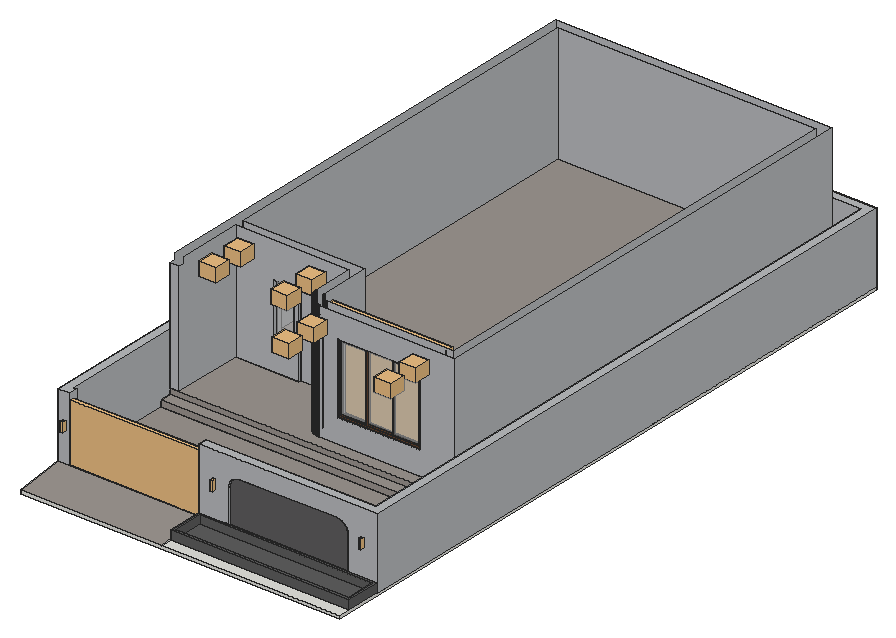
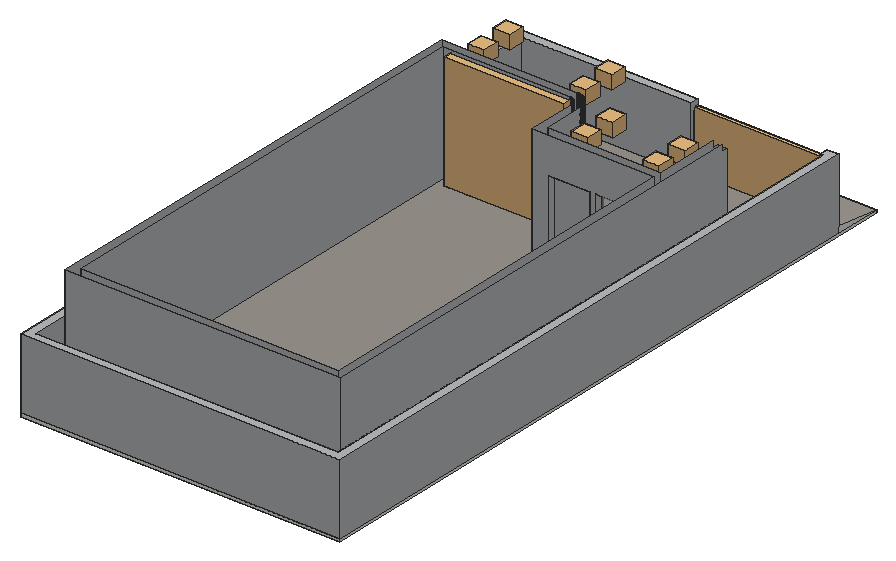
# SketchUp Ruby script. Lengths in inches.
U = 1.inch
M = Sketchup.active_model
def pt(a) = Geom::Point3d.new(a.map { |v| v * U })
def face(e, loops, mat)
  f = e.add_face(loops[0].map { |a| pt(a) })
  loops[1..].each { |l| e.add_face(l.map { |a| pt(a) }).erase! }
  f.material = f.back_material = mat if mat
  f
end
# faces: each face lists its corners as indices into pts; further lists are holes
def faces(e, pts, list, mat = nil) = list.each { |f| face(e, (f[0].is_a?(Array) ? f : [f]).map { |l| l.map { |i| pts[i] } }, mat) }
# xy, xz, yz: faces in a plane at the given z, y or x. An outline is a flat list of corners, or four numbers for a rectangle; further outlines are holes
def ring(l) = l.size == 4 ? [[l[0], l[1]], [l[2], l[1]], [l[2], l[3]], [l[0], l[3]]] : l.each_slice(2).to_a
def flat(e, list, mat, &to3) = list.each { |f| face(e, (f[0].is_a?(Array) ? f : [f]).map { |l| ring(l).map { |u, v| to3.(u, v) } }, mat) }
def xy(e, z, list, mat = nil) = flat(e, list, mat) { |x, y| [x, y, z] }
def xz(e, y, list, mat = nil) = flat(e, list, mat) { |x, z| [x, y, z] }
def yz(e, x, list, mat = nil) = flat(e, list, mat) { |y, z| [x, y, z] }
def lines(e, pts, list) = list.each { |a, b| e.add_line(pt(pts[a]), pt(pts[b])) }
# prism: a flat outline (further loops are holes) pulled along v
def prism(e, loops, v, mat = nil)
  f = face(e, loops, mat); d = Geom::Vector3d.new(v.map { |x| x * U })
  f.pushpull(f.normal.samedirection?(d) ? d.length : -d.length)
end
def box(e, o, s, mat = nil) = prism(e, [[o, [o[0] + s[0], o[1], o[2]], [o[0] + s[0], o[1] + s[1], o[2]], [o[0], o[1] + s[1], o[2]]]], [0, 0, s[2]], mat)
def at(x, y, z, deg = 0) = Geom::Transformation.translation(pt([x, y, z])) * Geom::Transformation.rotation(ORIGIN, Z_AXIS, deg.degrees)
def axes(o, x, y, z) = Geom::Transformation.new([*x, 0, *y, 0, *z, 0, *pt(o).to_a, 1])
def part(name) = M.definitions.add(name)
# library, detail: a bought-in or finely detailed component or shape, given as its bounding box
def library(name, o, s) = part(name).tap { |d| box(d.entities, o, s) }
def detail(e, o, s) = box(e.add_group.entities, o, s)
def put(e, d, t, mat = nil) = e.add_instance(d, t).tap { |i| i.material = mat if mat }
def group(e, t, mat = nil) = e.add_group.tap { |g| g.transformation = t; g.material = mat if mat }.entities
root = M.entities
M.materials.add("1422 AP 8231 MUTED GREY").color = [95, 93, 94]
M.materials.add("1427 AP 686 ARMOUR-N").color = [184, 186, 189]
M.materials.add("[Concrete Block 8x8 Gray]").color = [94, 94, 94]
M.materials.add("[Granite Tile]").color = [155, 148, 143]
M.materials.add("[Granite Tile]1").color = [155, 148, 143]
M.materials.add("[Translucent Glass Gray]").color = [206, 206, 206]
M.materials["[Translucent Glass Gray]"].alpha = 0.35
M.materials.add("[Wood Veneer 01]").color = [99, 65, 43]
c1 = library("Gate",[-1,-3.25,0],[122,4.25,84])
c2 = library("WALL LIGHT 69\#1",[4.19,4.05,-8.39],[4.61,5.7,16.35])
c3 = part("DOOR12")
g1 = group(c3.entities,at(114.73,30.14,-0.51))
g2 = group(g1,at(0,0,0))
box(g2,[0,0,0],[36,0.5,77.7])
c4 = library("Curtains",[0,0,0],[121.73,8.19,117.22])
c5 = part("Group\#26")
box(c5.entities,[0,0,0],[25,0.47,67])
c6 = library("2",[-6.43,-6.43,-13.78],[16.84,16.84,13.78])
xy(root,0,[[9,180,9,672,290,672,290,192,151.78,192,151.57,192.01,151.35,192.01,150.91,192.03,150.7,192.05,150.48,192.0625,150.26,192.08,150.05,192.11,149.83,192.13,149.61,192.16,149.4,192.1875,149.18,192.22,148.97,192.26,148.76,192.29,148.54,192.34,148.12,192.42,147.9,192.47,147.69,192.52,147.48,192.58,147.27,192.63,147.0625,192.69,146.85,192.75,146.64,192.82,146.4375,192.88,146.23,192.95,146.03,193.02,145.82,193.09,145.62,193.17,145.41,193.25,145.01,193.41,144.8125,193.5,144.61,193.59,144.41,193.68,144.22,193.77,144.02,193.86,143.83,193.96,143.63,194.0625,143.44,194.16,143.25,194.27,142.875,194.48,142.6875,194.6,142.5,194.71,142.32,194.83,142.14,194.94,141.95,195.0625,141.77,195.1875,141.6,195.3125,141.42,195.4375,141.24,195.57,140.9,195.83,140.73,195.97,140.56,196.1,140.39,196.24,140.23,196.38,140.0625,196.53,139.9,196.67,139.58,196.97,139.43,197.12,139.27,197.27,139.12,197.43,138.97,197.58,138.67,197.9,138.53,198.0625,138.38,198.23,138.24,198.39,138.1,198.56,137.97,198.73,137.83,198.9,137.57,199.24,137.4375,199.42,137.3125,199.6,137.1875,199.77,137.0625,199.95,136.94,200.14,136.83,200.32,136.71,200.5,136.6,200.6875,136.48,200.875,136.27,201.25,136.16,201.44,136.0625,201.63,135.96,201.83,135.86,202.02,135.77,202.22,135.68,202.41,135.59,202.61,135.5,202.8125,135.41,203.01,135.25,203.41,135.17,203.62,135.09,203.82,135.02,204.03,134.95,204.23,134.88,204.4375,134.82,204.64,134.75,204.85,134.69,205.0625,134.63,205.27,134.58,205.48,134.52,205.69,134.47,205.9,134.42,206.12,134.34,206.54,134.29,206.76,134.26,206.97,134.22,207.18,134.1875,207.4,134.16,207.61,134.13,207.83,134.11,208.05,134.08,208.26,134.0625,208.48,134.05,208.7,134.03,208.91,134.01,209.35,134.01,209.57,134,209.78,134,252,125,252,125,261,143,261,143,209.78,143.01,209.67,143.01,209.57,143.02,209.46,143.02,209.35,143.05,209.02,143.07,208.92,143.09,208.7,143.13,208.48,143.15,208.38,143.17,208.27,143.1875,208.16,143.21,208.06,143.24,207.95,143.26,207.85,143.29,207.74,143.32,207.64,143.35,207.53,143.375,207.43,143.41,207.32,143.47,207.12,143.51,207.01,143.55,206.91,143.58,206.81,143.625,206.71,143.66,206.61,143.71,206.51,143.79,206.31,143.84,206.21,143.88,206.11,143.98,205.91,144.03,205.82,144.08,205.72,144.13,205.625,144.1875,205.53,144.24,205.4375,144.3,205.34,144.35,205.25,144.59,204.89,144.66,204.8,144.78,204.62,144.85,204.54,144.92,204.45,144.98,204.36,145.12,204.2,145.19,204.11,145.26,204.03,145.34,203.95,145.48,203.79,145.56,203.71,145.64,203.64,145.71,203.56,145.79,203.48,145.95,203.34,146.03,203.26,146.11,203.19,146.2,203.12,146.36,202.98,146.45,202.92,146.54,202.85,146.62,202.78,146.8,202.66,146.89,202.59,147.25,202.35,147.34,202.3,147.4375,202.24,147.53,202.1875,147.625,202.13,147.72,202.08,147.82,202.03,147.91,201.98,148.11,201.88,148.21,201.84,148.31,201.79,148.51,201.71,148.61,201.66,148.71,201.625,148.81,201.58,148.91,201.55,149.01,201.51,149.12,201.47,149.32,201.41,149.43,201.375,149.53,201.35,149.64,201.32,149.74,201.29,149.85,201.26,149.95,201.24,150.06,201.21,150.16,201.1875,150.27,201.17,150.38,201.15,150.48,201.13,150.7,201.09,150.92,201.07,151.02,201.05,151.35,201.02,151.46,201.02,151.57,201.01,151.67,201.01,151.78,201,281,201,281,663,18,663,18,261,83,261,83,252,18,252,18,180]],"1427 AP 686 ARMOUR-N")
xy(root,24,[[170,192,254,201],[57,252,77,261]],"1427 AP 686 ARMOUR-N")
xy(root,84,[[57,252,77,261],[83,252,125,261]],"1427 AP 686 ARMOUR-N")
xy(root,96,[[170,192,254,201]],"1427 AP 686 ARMOUR-N")
xz(root,180,[[9,0,18,114]],"1427 AP 686 ARMOUR-N")
xz(root,192,[[151.78,0,152,120],[[152,0,290,120],[170,24,254,96]]],"1427 AP 686 ARMOUR-N")
xz(root,192.01,[[151.35,0,151.57,120]],"1427 AP 686 ARMOUR-N")
xz(root,201,[[151.78,0,151.89,120],[[151.89,0,281,120],[170,24,254,96]]],"1427 AP 686 ARMOUR-N")
xz(root,201.01,[[151.57,0,151.67,120]],"1427 AP 686 ARMOUR-N")
xz(root,201.02,[[151.35,0,151.46,120]],"1427 AP 686 ARMOUR-N")
xz(root,252,[[[18,0,83,0,83,84,125,84,125,0,134,0,134,120,18,120],[57,24,77,84]]],"1427 AP 686 ARMOUR-N")
xz(root,261,[[[18,0,18,120,143,120,143,0,125,0,125,84,83,84,83,0],[57,24,77,84]]],"1427 AP 686 ARMOUR-N")
xz(root,663,[[18,0,281,120]],"1427 AP 686 ARMOUR-N")
xz(root,672,[[9,0,290,120]],"1427 AP 686 ARMOUR-N")
yz(root,9,[[180,0,180,114,186,114,186,120,672,120,672,0]],"1427 AP 686 ARMOUR-N")
yz(root,18,[[180,0,252,0,252,120,186,120,186,114,180,114],[261,0,663,120]],"1427 AP 686 ARMOUR-N")
yz(root,57,[[252,24,261,84]],"1427 AP 686 ARMOUR-N")
yz(root,77,[[252,24,261,84]],"1427 AP 686 ARMOUR-N")
yz(root,83,[[252,0,261,84]],"1427 AP 686 ARMOUR-N")
yz(root,125,[[252,0,261,84]],"1427 AP 686 ARMOUR-N")
yz(root,134,[[209.78,0,210,120],[210,0,252,120]],"1427 AP 686 ARMOUR-N")
yz(root,134.01,[[209.35,0,209.57,120]],"1427 AP 686 ARMOUR-N")
yz(root,143,[[209.78,0,209.89,120],[209.89,0,261,120]],"1427 AP 686 ARMOUR-N")
yz(root,143.01,[[209.57,0,209.67,120]],"1427 AP 686 ARMOUR-N")
yz(root,143.02,[[209.35,0,209.46,120]],"1427 AP 686 ARMOUR-N")
yz(root,170,[[192,24,201,96]],"1427 AP 686 ARMOUR-N")
yz(root,254,[[192,24,201,96]],"1427 AP 686 ARMOUR-N")
yz(root,281,[[201,0,663,120]],"1427 AP 686 ARMOUR-N")
yz(root,290,[[192,0,672,120]],"1427 AP 686 ARMOUR-N")
p = [[150.7,192.05,120],[150.48,192.0625,120],[150.48,192.0625,0],[150.7,192.05,0],[150.91,192.03,120],[150.91,192.03,0],
  [151.13,192.02,120],[151.13,192.02,0],[151.35,192.01,120],[151.35,192.01,0],[151.78,192,120],[151.57,192.01,120],
  [151.57,192.01,0],[151.78,192,0],[149.83,192.13,120],[149.61,192.16,120],[149.61,192.16,0],[149.83,192.13,0],
  [150.05,192.11,120],[150.05,192.11,0],[150.26,192.08,120],[150.26,192.08,0],[149.18,192.22,120],[148.97,192.26,120],
  [148.97,192.26,0],[149.18,192.22,0],[149.4,192.1875,120],[149.4,192.1875,0],[148.54,192.34,120],[148.33,192.38,120],
  [148.33,192.38,0],[148.54,192.34,0],[148.76,192.29,120],[148.76,192.29,0],[148.12,192.42,120],[147.9,192.47,120],
  [147.9,192.47,0],[148.12,192.42,0],[147.69,192.52,120],[147.48,192.58,120],[147.48,192.58,0],[147.69,192.52,0],
  [147.27,192.63,120],[147.0625,192.69,120],[147.0625,192.69,0],[147.27,192.63,0],[146.85,192.75,120],[146.85,192.75,0],
  [146.64,192.82,120],[146.4375,192.88,120],[146.4375,192.88,0],[146.64,192.82,0],[146.23,192.95,120],[146.03,193.02,120],
  [146.03,193.02,0],[146.23,192.95,0],[145.82,193.09,120],[145.82,193.09,0],[145.62,193.17,120],[145.62,193.17,0],
  [145.41,193.25,120],[145.21,193.33,120],[145.21,193.33,0],[145.41,193.25,0],[145.01,193.41,120],[145.01,193.41,0],
  [144.8125,193.5,120],[144.8125,193.5,0],[144.61,193.59,120],[144.61,193.59,0],[144.41,193.68,120],[144.41,193.68,0],
  [144.22,193.77,120],[144.22,193.77,0],[144.02,193.86,120],[144.02,193.86,0],[143.83,193.96,120],[143.83,193.96,0],
  [143.63,194.0625,120],[143.63,194.0625,0],[143.44,194.16,120],[143.44,194.16,0],[143.25,194.27,120],[143.25,194.27,0],
  [143.0625,194.375,120],[143.0625,194.375,0],[142.875,194.48,120],[142.875,194.48,0],[142.6875,194.6,120],[142.6875,194.6,0],
  [142.5,194.71,120],[142.5,194.71,0],[142.32,194.83,120],[142.32,194.83,0],[142.14,194.94,120],[142.14,194.94,0],
  [141.95,195.0625,120],[141.95,195.0625,0],[141.77,195.1875,120],[141.77,195.1875,0],[141.6,195.3125,120],[141.6,195.3125,0],
  [141.42,195.4375,120],[141.42,195.4375,0],[141.24,195.57,120],[141.24,195.57,0],[141.07,195.7,120],[141.07,195.7,0],
  [140.9,195.83,120],[140.9,195.83,0],[140.73,195.97,120],[140.73,195.97,0],[140.56,196.1,120],[140.56,196.1,0],
  [140.39,196.24,120],[140.39,196.24,0],[140.23,196.38,120],[140.23,196.38,0],[140.0625,196.53,120],[140.0625,196.53,0],
  [139.9,196.67,120],[139.9,196.67,0],[139.74,196.82,120],[139.74,196.82,0],[139.58,196.97,120],[139.58,196.97,0],
  [139.43,197.12,120],[139.43,197.12,0],[139.27,197.27,120],[139.27,197.27,0],[139.12,197.43,120],[139.12,197.43,0],
  [138.97,197.58,120],[138.97,197.58,0],[138.82,197.74,120],[138.82,197.74,0],[138.67,197.9,120],[138.67,197.9,0],
  [138.53,198.0625,120],[138.53,198.0625,0],[138.38,198.23,120],[138.38,198.23,0],[138.24,198.39,120],[138.24,198.39,0],
  [138.1,198.56,120],[138.1,198.56,0],[137.97,198.73,120],[137.97,198.73,0],[137.83,198.9,120],[137.83,198.9,0],
  [137.7,199.07,120],[137.7,199.07,0],[137.57,199.24,120],[137.57,199.24,0],[137.4375,199.42,120],[137.4375,199.42,0],
  [137.3125,199.6,120],[137.3125,199.6,0],[137.1875,199.77,120],[137.1875,199.77,0],[137.0625,199.95,120],[137.0625,199.95,0],
  [136.94,200.14,120],[136.94,200.14,0],[136.83,200.32,120],[136.83,200.32,0],[136.71,200.5,120],[136.71,200.5,0],
  [136.6,200.6875,120],[136.6,200.6875,0],[136.48,200.875,120],[136.48,200.875,0],[136.375,201.0625,120],[136.375,201.0625,0],
  [151.02,201.05,120],[151.13,201.04,120],[151.13,201.04,0],[151.02,201.05,0],[151.24,201.03,120],[151.24,201.03,0],
  [151.35,201.02,120],[151.35,201.02,0],[151.46,201.02,120],[151.57,201.01,120],[151.57,201.01,0],[151.46,201.02,0],
  [151.67,201.01,120],[151.78,201,120],[151.78,201,0],[151.67,201.01,0],[136.27,201.25,120],[136.27,201.25,0],
  [150.27,201.17,120],[150.38,201.15,120],[150.38,201.15,0],[150.27,201.17,0],[150.48,201.13,120],[150.48,201.13,0],
  [150.59,201.11,120],[150.59,201.11,0],[150.7,201.09,120],[150.7,201.09,0],[150.81,201.08,120],[150.81,201.08,0],
  [150.92,201.07,120],[150.92,201.07,0],[149.85,201.26,120],[149.95,201.24,120],[149.95,201.24,0],[149.85,201.26,0],
  [150.06,201.21,120],[150.06,201.21,0],[150.16,201.1875,120],[150.16,201.1875,0],[136.16,201.44,120],[136.16,201.44,0],
  [149.43,201.375,120],[149.53,201.35,120],[149.53,201.35,0],[149.43,201.375,0],[149.64,201.32,120],[149.64,201.32,0],
  [149.74,201.29,120],[149.74,201.29,0],[136.0625,201.63,120],[136.0625,201.63,0],[149.12,201.47,120],[149.22,201.44,120],
  [149.22,201.44,0],[149.12,201.47,0],[149.32,201.41,120],[149.32,201.41,0],[148.81,201.58,120],[148.91,201.55,120],
  [148.91,201.55,0],[148.81,201.58,0],[149.01,201.51,120],[149.01,201.51,0],[135.96,201.83,120],[135.96,201.83,0],
  [148.61,201.66,120],[148.71,201.625,120],[148.71,201.625,0],[148.61,201.66,0],[148.31,201.79,120],[148.41,201.75,120],
  [148.41,201.75,0],[148.31,201.79,0],[148.51,201.71,120],[148.51,201.71,0],[135.86,202.02,120],[135.86,202.02,0],
  [148.11,201.88,120],[148.21,201.84,120],[148.21,201.84,0],[148.11,201.88,0],[147.91,201.98,120],[148.01,201.93,120],
  [148.01,201.93,0],[147.91,201.98,0],[135.77,202.22,120],[135.77,202.22,0],[147.72,202.08,120],[147.82,202.03,120],
  [147.82,202.03,0],[147.72,202.08,0],[147.53,202.1875,120],[147.625,202.13,120],[147.625,202.13,0],[147.53,202.1875,0],
  [135.68,202.41,120],[135.68,202.41,0],[147.34,202.3,120],[147.4375,202.24,120],[147.4375,202.24,0],[147.34,202.3,0],
  [147.25,202.35,120],[147.25,202.35,0],[135.59,202.61,120],[135.59,202.61,0],[147.07,202.47,120],[147.16,202.41,120],
  [147.16,202.41,0],[147.07,202.47,0],[146.89,202.59,120],[146.98,202.53,120],[146.98,202.53,0],[146.89,202.59,0],
  [135.5,202.8125,120],[135.5,202.8125,0],[146.8,202.66,120],[146.8,202.66,0],[146.62,202.78,120],[146.71,202.72,120],
  [146.71,202.72,0],[146.62,202.78,0],[135.41,203.01,120],[135.41,203.01,0],[146.45,202.92,120],[146.54,202.85,120],
  [146.54,202.85,0],[146.45,202.92,0],[146.36,202.98,120],[146.36,202.98,0],[135.33,203.21,120],[135.33,203.21,0],
  [146.28,203.05,120],[146.28,203.05,0],[146.11,203.19,120],[146.2,203.12,120],[146.2,203.12,0],[146.11,203.19,0],
  [135.25,203.41,120],[135.25,203.41,0],[146.03,203.26,120],[146.03,203.26,0],[145.87,203.41,120],[145.95,203.34,120],
  [145.95,203.34,0],[145.87,203.41,0],[135.17,203.62,120],[135.17,203.62,0],[145.79,203.48,120],[145.79,203.48,0],
  [145.71,203.56,120],[145.71,203.56,0],[135.09,203.82,120],[135.09,203.82,0],[145.64,203.64,120],[145.64,203.64,0],
  [145.56,203.71,120],[145.56,203.71,0],[145.48,203.79,120],[145.48,203.79,0],[135.02,204.03,120],[135.02,204.03,0],
  [145.41,203.87,120],[145.41,203.87,0],[145.34,203.95,120],[145.34,203.95,0],[134.95,204.23,120],[134.95,204.23,0],
  [145.19,204.11,120],[145.26,204.03,120],[145.26,204.03,0],[145.19,204.11,0],[145.12,204.2,120],[145.12,204.2,0],
  [134.88,204.4375,120],[134.88,204.4375,0],[145.05,204.28,120],[145.05,204.28,0],[144.98,204.36,120],[144.98,204.36,0],
  [134.82,204.64,120],[134.82,204.64,0],[144.85,204.54,120],[144.92,204.45,120],[144.92,204.45,0],[144.85,204.54,0],
  [144.78,204.62,120],[144.78,204.62,0],[134.75,204.85,120],[134.75,204.85,0],[144.72,204.71,120],[144.72,204.71,0],
  [144.66,204.8,120],[144.66,204.8,0],[144.59,204.89,120],[144.59,204.89,0],[134.69,205.0625,120],[134.69,205.0625,0],
  [144.53,204.98,120],[144.53,204.98,0],[144.47,205.07,120],[144.47,205.07,0],[134.63,205.27,120],[134.63,205.27,0],
  [144.41,205.16,120],[144.41,205.16,0],[144.35,205.25,120],[144.35,205.25,0],[134.58,205.48,120],[134.58,205.48,0],
  [144.24,205.4375,120],[144.3,205.34,120],[144.3,205.34,0],[144.24,205.4375,0],[144.1875,205.53,120],[144.1875,205.53,0],
  [134.52,205.69,120],[134.52,205.69,0],[144.13,205.625,120],[144.13,205.625,0],[144.08,205.72,120],[144.08,205.72,0],
  [134.47,205.9,120],[134.47,205.9,0],[144.03,205.82,120],[144.03,205.82,0],[143.98,205.91,120],[143.98,205.91,0],
  [134.42,206.12,120],[134.42,206.12,0],[143.93,206.01,120],[143.93,206.01,0],[143.88,206.11,120],[143.88,206.11,0],
  [134.38,206.33,120],[134.38,206.33,0],[143.84,206.21,120],[143.84,206.21,0],[143.79,206.31,120],[143.79,206.31,0],
  [134.34,206.54,120],[134.34,206.54,0],[143.75,206.41,120],[143.75,206.41,0],[143.71,206.51,120],[143.71,206.51,0],
  [134.29,206.76,120],[134.29,206.76,0],[143.66,206.61,120],[143.66,206.61,0],[143.625,206.71,120],[143.625,206.71,0],
  [143.58,206.81,120],[143.58,206.81,0],[134.26,206.97,120],[134.26,206.97,0],[143.55,206.91,120],[143.55,206.91,0],
  [143.51,207.01,120],[143.51,207.01,0],[134.22,207.18,120],[134.22,207.18,0],[143.47,207.12,120],[143.47,207.12,0],
  [143.44,207.22,120],[143.44,207.22,0],[134.1875,207.4,120],[134.1875,207.4,0],[143.41,207.32,120],[143.41,207.32,0],
  [143.375,207.43,120],[143.375,207.43,0],[134.16,207.61,120],[134.16,207.61,0],[143.35,207.53,120],[143.35,207.53,0],
  [143.32,207.64,120],[143.32,207.64,0],[134.13,207.83,120],[134.13,207.83,0],[143.29,207.74,120],[143.29,207.74,0],
  [143.26,207.85,120],[143.26,207.85,0],[134.11,208.05,120],[134.11,208.05,0],[143.24,207.95,120],[143.24,207.95,0],
  [134.08,208.26,120],[134.08,208.26,0],[143.21,208.06,120],[143.21,208.06,0],[143.1875,208.16,120],[143.1875,208.16,0],
  [143.17,208.27,120],[143.17,208.27,0],[134.0625,208.48,120],[134.0625,208.48,0],[143.15,208.38,120],[143.15,208.38,0],
  [143.13,208.48,120],[143.13,208.48,0],[134.05,208.7,120],[134.05,208.7,0],[143.11,208.59,120],[143.11,208.59,0],
  [143.09,208.7,120],[143.09,208.7,0],[134.03,208.91,120],[134.03,208.91,0],[143.08,208.81,120],[143.08,208.81,0],
  [143.07,208.92,120],[143.07,208.92,0],[134.02,209.13,120],[134.02,209.13,0],[143.05,209.02,120],[143.05,209.02,0],
  [143.04,209.13,120],[143.04,209.13,0],[134.01,209.35,120],[134.01,209.35,0],[143.03,209.24,120],[143.03,209.24,0],
  [143.02,209.35,120],[143.02,209.35,0],[143.01,209.57,120],[143.02,209.46,120],[143.02,209.46,0],[143.01,209.57,0],
  [134.01,209.57,120],[134,209.78,120],[134,209.78,0],[134.01,209.57,0],[143,209.78,120],[143.01,209.67,120],
  [143.01,209.67,0],[143,209.78,0]]
faces(root,p,[[0,1,2,3],[4,0,3,5],[6,4,5,7],[8,6,7,9],[10,11,12,13],[14,15,16,17],[18,14,17,19],[20,18,19,21],
  [1,20,21,2],[22,23,24,25],[26,22,25,27],[15,26,27,16],[28,29,30,31],[32,28,31,33],[23,32,33,24],[34,35,36,37],
  [29,34,37,30],[38,39,40,41],[35,38,41,36],[42,43,44,45],[39,42,45,40],[43,46,47,44],[48,49,50,51],[46,48,51,47],
  [52,53,54,55],[49,52,55,50],[53,56,57,54],[56,58,59,57],[60,61,62,63],[58,60,63,59],[61,64,65,62],[64,66,67,65],
  [66,68,69,67],[68,70,71,69],[70,72,73,71],[72,74,75,73],[74,76,77,75],[76,78,79,77],[78,80,81,79],[80,82,83,81],
  [82,84,85,83],[84,86,87,85],[86,88,89,87],[88,90,91,89],[90,92,93,91],[92,94,95,93],[94,96,97,95],[96,98,99,97],
  [98,100,101,99],[100,102,103,101],[102,104,105,103],[104,106,107,105],[106,108,109,107],[108,110,111,109],[110,112,113,111],[112,114,115,113],
  [114,116,117,115],[116,118,119,117],[118,120,121,119],[120,122,123,121],[122,124,125,123],[124,126,127,125],[126,128,129,127],[128,130,131,129],
  [130,132,133,131],[132,134,135,133],[134,136,137,135],[136,138,139,137],[138,140,141,139],[140,142,143,141],[142,144,145,143],[144,146,147,145],
  [146,148,149,147],[148,150,151,149],[150,152,153,151],[152,154,155,153],[154,156,157,155],[156,158,159,157],[158,160,161,159],[160,162,163,161],
  [162,164,165,163],[164,166,167,165],[166,168,169,167],[168,170,171,169],[170,172,173,171],[174,175,176,177],[175,178,179,176],[178,180,181,179],
  [182,183,184,185],[186,187,188,189],[172,190,191,173],[192,193,194,195],[193,196,197,194],[196,198,199,197],[198,200,201,199],[200,202,203,201],
  [202,204,205,203],[204,174,177,205],[206,207,208,209],[207,210,211,208],[210,212,213,211],[212,192,195,213],[190,214,215,191],[216,217,218,219],
  [217,220,221,218],[220,222,223,221],[222,206,209,223],[214,224,225,215],[226,227,228,229],[227,230,231,228],[230,216,219,231],[232,233,234,235],
  [233,236,237,234],[236,226,229,237],[224,238,239,225],[240,241,242,243],[241,232,235,242],[244,245,246,247],[245,248,249,246],[248,240,243,249],
  [238,250,251,239],[252,253,254,255],[253,244,247,254],[256,257,258,259],[257,252,255,258],[250,260,261,251],[262,263,264,265],[263,256,259,264],
  [266,267,268,269],[267,262,265,268],[260,270,271,261],[272,273,274,275],[273,266,269,274],[276,272,275,277],[270,278,279,271],[280,281,282,283],
  [281,276,277,282],[284,285,286,287],[285,280,283,286],[278,288,289,279],[290,284,287,291],[292,293,294,295],[293,290,291,294],[288,296,297,289],
  [298,299,300,301],[299,292,295,300],[302,298,301,303],[296,304,305,297],[306,302,303,307],[308,309,310,311],[309,306,307,310],[304,312,313,305],
  [314,308,311,315],[316,317,318,319],[317,314,315,318],[312,320,321,313],[322,316,319,323],[324,322,323,325],[320,326,327,321],[328,324,325,329],
  [330,328,329,331],[332,330,331,333],[326,334,335,327],[336,332,333,337],[338,336,337,339],[334,340,341,335],[342,343,344,345],[343,338,339,344],
  [346,342,345,347],[340,348,349,341],[350,346,347,351],[352,350,351,353],[348,354,355,349],[356,357,358,359],[357,352,353,358],[360,356,359,361],
  [354,362,363,355],[364,360,361,365],[366,364,365,367],[368,366,367,369],[362,370,371,363],[372,368,369,373],[374,372,373,375],[370,376,377,371],
  [378,374,375,379],[380,378,379,381],[376,382,383,377],[384,385,386,387],[385,380,381,386],[388,384,387,389],[382,390,391,383],[392,388,389,393],
  [394,392,393,395],[390,396,397,391],[398,394,395,399],[400,398,399,401],[396,402,403,397],[404,400,401,405],[406,404,405,407],[402,408,409,403],
  [410,406,407,411],[412,410,411,413],[408,414,415,409],[416,412,413,417],[418,416,417,419],[414,420,421,415],[422,418,419,423],[424,422,423,425],
  [426,424,425,427],[420,428,429,421],[430,426,427,431],[432,430,431,433],[428,434,435,429],[436,432,433,437],[438,436,437,439],[434,440,441,435],
  [442,438,439,443],[444,442,443,445],[440,446,447,441],[448,444,445,449],[450,448,449,451],[446,452,453,447],[454,450,451,455],[456,454,455,457],
  [452,458,459,453],[460,456,457,461],[458,462,463,459],[464,460,461,465],[466,464,465,467],[468,466,467,469],[462,470,471,463],[472,468,469,473],
  [474,472,473,475],[470,476,477,471],[478,474,475,479],[480,478,479,481],[476,482,483,477],[484,480,481,485],[486,484,485,487],[482,488,489,483],
  [490,486,487,491],[492,490,491,493],[488,494,495,489],[496,492,493,497],[498,496,497,499],[500,501,502,503],[504,505,506,507],[508,509,510,511]],"1427 AP 686 ARMOUR-N")
g3 = group(root,at(0,11.98,-18))
box(g3,[0,-11.98,-3],[326,684,3])
g4 = group(root,at(11.89,48,-18))
xy(g4,0,[[-11.89,-48,132.11,0]])
xz(g4,0,[[-11.89,0,132.11,6]])
yz(g4,-11.89,[[-48,0,0,6,0,0]])
yz(g4,132.11,[[-48,0,0,0,0,6]])
p = [[132.11,0,6],[-11.89,0,6],[-11.89,-48,0],[132.11,-48,0]]
faces(g4,p,[[0,1,2,3]],"[Granite Tile]1")
g5 = group(root,at(9,168,-12),"1427 AP 686 ARMOUR-N")
xy(g5,-6,[[-9,-120,-9,516,317,516,317,-120,287,-120,287,-118,165,-118,165,-120],[165,-120,287,-118]])
xy(g5,0,[[3,-120,135,-120,135,-111,308,-111,308,507,0,507,0,-111,3,-111]],"[Granite Tile]")
xy(g5,48,[[177,-120,275,-118]])
xy(g5,66,[[-9,-120,3,-120,3,-111,0,-111,0,507,308,507,308,-111,135,-111,135,-120,317,-120,317,516,-9,516]])
xz(g5,-120,[[-9,-6,165,-6,165,36,165.1,37.57,165.41,39.11,165.91,40.59,166.61,42,167.48,43.31,168.51,44.49,169.69,45.52,171,46.39,172.41,47.09,173.89,47.59,175.43,47.9,177,48,275,48,276.57,47.9,278.11,47.59,279.59,47.09,281,46.39,282.31,45.52,283.49,44.49,284.52,43.31,285.39,42,286.09,40.59,286.59,39.11,286.9,37.57,287,36,287,-6,317,-6,317,66,135,66,135,0,3,0,3,66,-9,66]])
xz(g5,-118,[[165,-6,287,-6,287,36,286.9,37.57,286.59,39.11,286.09,40.59,285.39,42,284.52,43.31,283.49,44.49,282.31,45.52,281,46.39,279.59,47.09,278.11,47.59,276.57,47.9,275,48,177,48,175.43,47.9,173.89,47.59,172.41,47.09,171,46.39,169.69,45.52,168.51,44.49,167.48,43.31,166.61,42,165.91,40.59,165.41,39.11,165.1,37.57,165,36]],"1422 AP 8231 MUTED GREY")
xz(g5,-111,[[0,0,3,66],[135,0,308,66]])
xz(g5,507,[[0,0,308,66]])
xz(g5,516,[[-9,-6,317,66]])
yz(g5,-9,[[-120,-6,516,66]])
yz(g5,0,[[-111,0,507,66]])
yz(g5,3,[[-120,0,-111,66]])
yz(g5,135,[[-120,0,-111,66]])
yz(g5,165,[[-120,-6,-118,36]])
yz(g5,287,[[-120,-6,-118,36]])
yz(g5,308,[[-111,0,507,66]])
yz(g5,317,[[-120,-6,516,66]])
p = [[165.1,-120,37.57],[165,-120,36],[165,-118,36],[165.1,-118,37.57],[287,-120,36],[286.9,-120,37.57],
  [286.9,-118,37.57],[287,-118,36],[165.41,-120,39.11],[165.41,-118,39.11],[286.59,-120,39.11],[286.59,-118,39.11],
  [165.91,-120,40.59],[165.91,-118,40.59],[286.09,-120,40.59],[286.09,-118,40.59],[166.61,-120,42],[166.61,-118,42],
  [285.39,-120,42],[285.39,-118,42],[167.48,-120,43.31],[167.48,-118,43.31],[284.52,-120,43.31],[284.52,-118,43.31],
  [168.51,-120,44.49],[168.51,-118,44.49],[283.49,-120,44.49],[283.49,-118,44.49],[169.69,-120,45.52],[169.69,-118,45.52],
  [282.31,-120,45.52],[282.31,-118,45.52],[171,-120,46.39],[171,-118,46.39],[281,-120,46.39],[281,-118,46.39],
  [172.41,-120,47.09],[172.41,-118,47.09],[279.59,-120,47.09],[279.59,-118,47.09],[173.89,-120,47.59],[173.89,-118,47.59],
  [278.11,-120,47.59],[278.11,-118,47.59],[175.43,-120,47.9],[175.43,-118,47.9],[276.57,-120,47.9],[276.57,-118,47.9],
  [177,-120,48],[177,-118,48],[275,-120,48],[275,-118,48]]
faces(g5,p,[[0,1,2,3],[4,5,6,7],[8,0,3,9],[5,10,11,6],[12,8,9,13],[10,14,15,11],[16,12,13,17],[14,18,19,15],
  [20,16,17,21],[18,22,23,19],[24,20,21,25],[22,26,27,23],[28,24,25,29],[26,30,31,27],[32,28,29,33],[30,34,35,31],
  [36,32,33,37],[34,38,39,35],[40,36,37,41],[38,42,43,39],[44,40,41,45],[42,46,47,43],[48,44,45,49],[46,50,51,47]])
put(g5,c1,axes([4.08,-116.75,0],[1.08197,0,0],[0,1,0],[0,0,0.71429]))
put(g5,c2,axes([146.1,-125.85,34.51],[0.6,0,0],[0,0.6,0],[0,0,0.6]))
put(g5,c2,axes([297.66,-125.85,34.51],[0.6,0,0],[0,0.6,0],[0,0,0.6]))
put(g5,c2,axes([-6.58,-125.85,34.51],[0.6,0,0],[0,0.6,0],[0,0,0.6]))
g6 = group(g5,at(135,-137.27,-6),"[Concrete Block 8x8 Gray]")
xy(g6,0,[[0,-18.75,182,17.27]])
xy(g6,1,[[3,-15.75,179,14.27]])
xy(g6,9,[[[0,-18.75,182,17.27],[3,-15.75,179,14.27]]])
xz(g6,-18.75,[[0,0,182,9]])
xz(g6,-15.75,[[3,1,179,9]])
xz(g6,14.27,[[3,1,179,9]])
xz(g6,17.27,[[0,0,30,9],[30,0,152,9],[152,0,182,9]])
yz(g6,0,[[-18.75,0,17.27,9]])
yz(g6,3,[[-15.75,1,14.27,9]])
yz(g6,179,[[-15.75,1,14.27,9]])
yz(g6,182,[[-18.75,0,17.27,9]])
g7 = group(root,at(9,192,-6),"[Granite Tile]")
box(g7,[0,-24,-6],[281,504,6])
g8 = group(root,at(9,192,0),"[Granite Tile]")
box(g8,[0,-12,-6],[281,492,6])
put(root,c3,axes([-50.85,223.86,0.55],[1.16667,0,0],[0,1,0],[0,0,1.08111]),"1427 AP 686 ARMOUR-N")
put(root,c4,at(151.89,201,0),"1427 AP 686 ARMOUR-N")
g9 = group(root,at(57,254,24),"[Wood Veneer 01]")
prism(g9,[[[20,0,60],[0,0,60],[0,0,0],[20,0,0]],[[1,0,59],[19,0,59],[19,0,1],[1,0,1]]],[0,1,0])
g10 = group(g9,at(1,0.26,1))
box(g10,[0,0,0],[18,0.47,58],"[Translucent Glass Gray]")
g11 = group(root,at(170,196.5,24),"[Wood Veneer 01]")
prism(g11,[[[84,0,0],[0,0,0],[0,0,72],[84,0,72]],[[1.5,0,1.5],[82.5,0,1.5],[82.5,0,70.5],[1.5,0,70.5]]],[0,-3,0])
g12 = group(g11,at(1.5,-1.25,1.5))
prism(g12,[[[27,-0.5,0],[0,-0.5,0],[0,-0.5,69],[27,-0.5,69]],[[26,-0.5,1],[26,-0.5,68],[1,-0.5,68],[1,-0.5,1]]],[0,-1,0])
put(g12,c5,at(1,-1.25,1),"[Translucent Glass Gray]")
g13 = group(g11,at(28.5,-0.25,1.5))
prism(g13,[[[27,-0.5,0],[0,-0.5,0],[0,-0.5,69],[27,-0.5,69]],[[26,-0.5,1],[26,-0.5,68],[1,-0.5,68],[1,-0.5,1]]],[0,-1,0])
put(g13,c5,at(1,-1.25,1),"[Translucent Glass Gray]")
g14 = group(g11,at(55.5,-1.5,1.5))
prism(g14,[[[27,-0.5,0],[0,-0.5,0],[0,-0.5,69],[27,-0.5,69]],[[26,-0.5,1],[26,-0.5,68],[1,-0.5,68],[1,-0.5,1]]],[0,-1,0])
put(g14,c5,at(1,-1.25,1),"[Translucent Glass Gray]")
put(root,c6,at(158.01,138.01,117.5))
put(root,c6,at(158.01,170.01,117.5))
put(root,c6,at(262.01,170.01,117.5))
put(root,c6,at(262.01,138.01,117.5))
put(root,c6,at(108.51,198.01,117.5))
put(root,c6,at(108.51,230.01,117.5))
put(root,c6,at(35.51,230.01,117.5))
put(root,c6,at(35.51,198.01,117.5))
